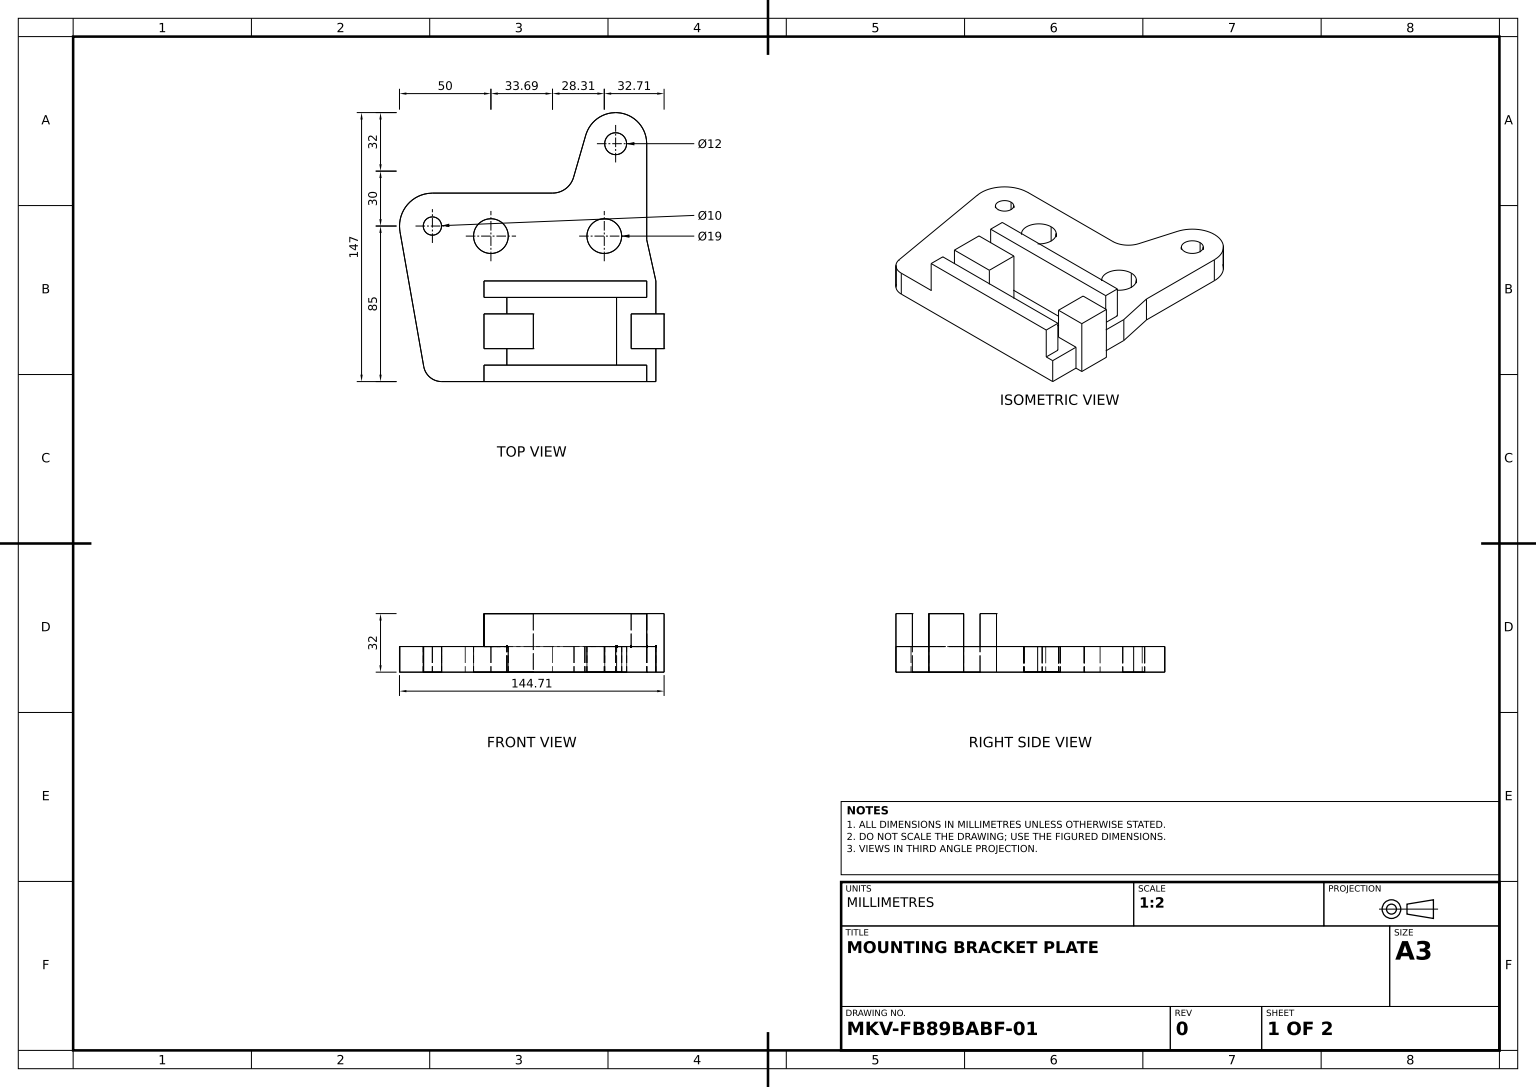
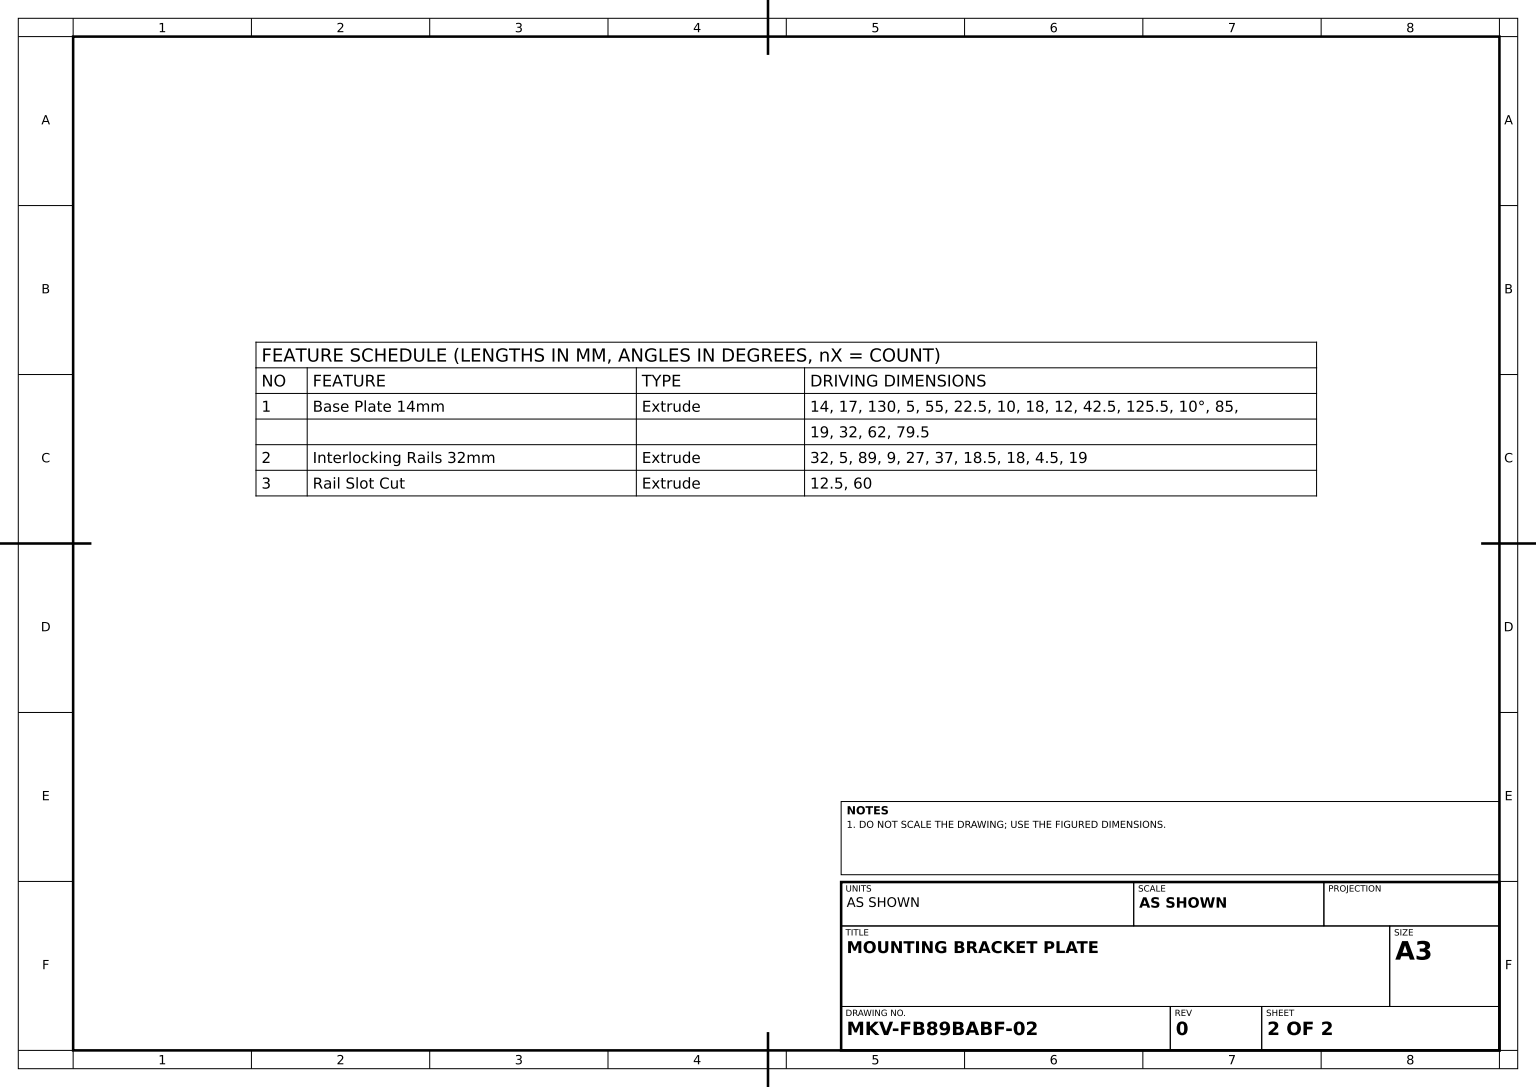
ISO-10303-21;
HEADER;
FILE_DESCRIPTION((''),'2;1');
FILE_NAME('','',(''),(''),'','','');
FILE_SCHEMA(('AUTOMOTIVE_DESIGN'));
ENDSEC;
DATA;
#1=APPLICATION_CONTEXT('');
#2=PRODUCT_CONTEXT('',#1,'mechanical');
#3=PRODUCT('','','',(#2));
#4=PRODUCT_DEFINITION_FORMATION('','',#3);
#5=PRODUCT_DEFINITION_CONTEXT('',#1,'design');
#6=PRODUCT_DEFINITION('','',#4,#5);
#7=PRODUCT_DEFINITION_SHAPE('','',#6);
#8=(LENGTH_UNIT()NAMED_UNIT(*)SI_UNIT(.MILLI.,.METRE.));
#9=(NAMED_UNIT(*)PLANE_ANGLE_UNIT()SI_UNIT($,.RADIAN.));
#10=(NAMED_UNIT(*)SI_UNIT($,.STERADIAN.)SOLID_ANGLE_UNIT());
#11=UNCERTAINTY_MEASURE_WITH_UNIT(LENGTH_MEASURE(1.E-05),#8,'distance_accuracy_value','');
#12=(GEOMETRIC_REPRESENTATION_CONTEXT(3)GLOBAL_UNCERTAINTY_ASSIGNED_CONTEXT((#11))GLOBAL_UNIT_ASSIGNED_CONTEXT((#8,#9,#10))REPRESENTATION_CONTEXT('',''));
#13=CARTESIAN_POINT('',(-67.,32.,-37.));
#14=VERTEX_POINT('',#13);
#15=CARTESIAN_POINT('',(-67.,0.,-37.));
#16=VERTEX_POINT('',#15);
#17=DIRECTION('',(0.,-1.,0.));
#18=VECTOR('',#17,1000.);
#19=LINE('',#13,#18);
#20=EDGE_CURVE('',#14,#16,#19,.T.);
#21=ORIENTED_EDGE('',*,*,#20,.T.);
#22=CARTESIAN_POINT('',(-81.5,0.,-37.));
#23=VERTEX_POINT('',#22);
#24=DIRECTION('',(-1.,0.,0.));
#25=VECTOR('',#24,1000.);
#26=LINE('',#15,#25);
#27=EDGE_CURVE('',#16,#23,#26,.T.);
#28=ORIENTED_EDGE('',*,*,#27,.T.);
#29=CARTESIAN_POINT('',(-81.5,14.,-37.));
#30=VERTEX_POINT('',#29);
#31=CARTESIAN_POINT('',(-81.5,-0.001,-37.));
#32=DIRECTION('',(0.,1.,0.));
#33=VECTOR('',#32,1000.);
#34=LINE('',#31,#33);
#35=EDGE_CURVE('',#23,#30,#34,.T.);
#36=ORIENTED_EDGE('',*,*,#35,.T.);
#37=CARTESIAN_POINT('',(-94.,14.,-37.));
#38=VERTEX_POINT('',#37);
#39=CARTESIAN_POINT('',(-22.,14.,-37.));
#40=DIRECTION('',(1.,0.,0.));
#41=VECTOR('',#40,1000.);
#42=LINE('',#39,#41);
#43=EDGE_CURVE('',#38,#30,#42,.T.);
#44=ORIENTED_EDGE('',*,*,#43,.F.);
#45=CARTESIAN_POINT('',(-94.,32.,-37.));
#46=VERTEX_POINT('',#45);
#47=LINE('',#45,#18);
#48=EDGE_CURVE('',#46,#38,#47,.T.);
#49=ORIENTED_EDGE('',*,*,#48,.F.);
#50=LINE('',#45,#25);
#51=EDGE_CURVE('',#14,#46,#50,.T.);
#52=ORIENTED_EDGE('',*,*,#51,.F.);
#53=EDGE_LOOP('',(#21,#28,#36,#44,#49,#52));
#54=FACE_OUTER_BOUND('',#53,.T.);
#55=DIRECTION('',(0.,0.,1.));
#56=AXIS2_PLACEMENT_3D('',#45,#55,#40);
#57=PLANE('',#56);
#58=ADVANCED_FACE('',(#54),#57,.F.);
#59=CARTESIAN_POINT('',(-22.,14.,-124.));
#60=VERTEX_POINT('',#59);
#61=CARTESIAN_POINT('',(-22.,14.,-136.));
#62=VERTEX_POINT('',#61);
#63=CARTESIAN_POINT('',(-22.,14.,-130.));
#64=AXIS2_PLACEMENT_3D('',#63,#32,#55);
#65=CIRCLE('',#64,6.);
#66=EDGE_CURVE('',#60,#62,#65,.T.);
#67=ORIENTED_EDGE('',*,*,#66,.T.);
#68=CARTESIAN_POINT('',(-22.,0.,-136.));
#69=VERTEX_POINT('',#68);
#70=LINE('',#61,#18);
#71=EDGE_CURVE('',#62,#69,#70,.T.);
#72=ORIENTED_EDGE('',*,*,#71,.T.);
#73=CARTESIAN_POINT('',(-22.,0.,-124.));
#74=VERTEX_POINT('',#73);
#75=CARTESIAN_POINT('',(-22.,0.,-130.));
#76=AXIS2_PLACEMENT_3D('',#75,#32,#55);
#77=CIRCLE('',#76,6.);
#78=EDGE_CURVE('',#74,#69,#77,.T.);
#79=ORIENTED_EDGE('',*,*,#78,.F.);
#80=LINE('',#59,#18);
#81=EDGE_CURVE('',#60,#74,#80,.T.);
#82=ORIENTED_EDGE('',*,*,#81,.F.);
#83=EDGE_LOOP('',(#67,#72,#79,#82));
#84=FACE_OUTER_BOUND('',#83,.T.);
#85=DIRECTION('',(0.,0.,-1.));
#86=AXIS2_PLACEMENT_3D('',#63,#17,#85);
#87=CYLINDRICAL_SURFACE('',#86,6.);
#88=ADVANCED_FACE('',(#84),#87,.F.);
#89=ORIENTED_EDGE('',*,*,#20,.F.);
#90=CARTESIAN_POINT('',(-67.,32.,-18.));
#91=VERTEX_POINT('',#90);
#92=VECTOR('',#85,1000.);
#93=LINE('',#90,#92);
#94=EDGE_CURVE('',#91,#14,#93,.T.);
#95=ORIENTED_EDGE('',*,*,#94,.F.);
#96=CARTESIAN_POINT('',(-67.,0.,-18.));
#97=VERTEX_POINT('',#96);
#98=LINE('',#90,#18);
#99=EDGE_CURVE('',#91,#97,#98,.T.);
#100=ORIENTED_EDGE('',*,*,#99,.T.);
#101=LINE('',#15,#92);
#102=EDGE_CURVE('',#97,#16,#101,.T.);
#103=ORIENTED_EDGE('',*,*,#102,.T.);
#104=EDGE_LOOP('',(#89,#95,#100,#103));
#105=FACE_OUTER_BOUND('',#104,.T.);
#106=AXIS2_PLACEMENT_3D('',#90,#24,#55);
#107=PLANE('',#106);
#108=ADVANCED_FACE('',(#105),#107,.F.);
#109=CARTESIAN_POINT('',(0.,14.,-18.));
#110=VERTEX_POINT('',#109);
#111=CARTESIAN_POINT('',(0.,0.,-18.));
#112=VERTEX_POINT('',#111);
#113=LINE('',#109,#18);
#114=EDGE_CURVE('',#110,#112,#113,.T.);
#115=ORIENTED_EDGE('',*,*,#114,.F.);
#116=CARTESIAN_POINT('',(0.,14.,0.));
#117=VERTEX_POINT('',#116);
#118=LINE('',#116,#92);
#119=EDGE_CURVE('',#117,#110,#118,.T.);
#120=ORIENTED_EDGE('',*,*,#119,.F.);
#121=CARTESIAN_POINT('',(0.,0.,0.));
#122=VERTEX_POINT('',#121);
#123=LINE('',#116,#18);
#124=EDGE_CURVE('',#117,#122,#123,.T.);
#125=ORIENTED_EDGE('',*,*,#124,.T.);
#126=LINE('',#121,#92);
#127=EDGE_CURVE('',#122,#112,#126,.T.);
#128=ORIENTED_EDGE('',*,*,#127,.T.);
#129=EDGE_LOOP('',(#115,#120,#125,#128));
#130=FACE_OUTER_BOUND('',#129,.T.);
#131=AXIS2_PLACEMENT_3D('',#116,#24,#55);
#132=PLANE('',#131);
#133=ADVANCED_FACE('',(#130),#132,.F.);
#134=CARTESIAN_POINT('',(-13.5,32.,-18.));
#135=VERTEX_POINT('',#134);
#136=CARTESIAN_POINT('',(4.5,32.,-18.));
#137=VERTEX_POINT('',#136);
#138=LINE('',#134,#41);
#139=EDGE_CURVE('',#135,#137,#138,.T.);
#140=ORIENTED_EDGE('',*,*,#139,.T.);
#141=CARTESIAN_POINT('',(4.5,32.,-37.));
#142=VERTEX_POINT('',#141);
#143=LINE('',#141,#92);
#144=EDGE_CURVE('',#137,#142,#143,.T.);
#145=ORIENTED_EDGE('',*,*,#144,.T.);
#146=CARTESIAN_POINT('',(-13.5,32.,-37.));
#147=VERTEX_POINT('',#146);
#148=LINE('',#146,#25);
#149=EDGE_CURVE('',#142,#147,#148,.T.);
#150=ORIENTED_EDGE('',*,*,#149,.T.);
#151=VECTOR('',#55,1000.);
#152=LINE('',#146,#151);
#153=EDGE_CURVE('',#147,#135,#152,.T.);
#154=ORIENTED_EDGE('',*,*,#153,.T.);
#155=EDGE_LOOP('',(#140,#145,#150,#154));
#156=FACE_OUTER_BOUND('',#155,.T.);
#157=CARTESIAN_POINT('',(0.,32.,0.));
#158=AXIS2_PLACEMENT_3D('',#157,#32,#55);
#159=PLANE('',#158);
#160=ADVANCED_FACE('',(#156),#159,.T.);
#161=ORIENTED_EDGE('',*,*,#48,.T.);
#162=CARTESIAN_POINT('',(-94.,14.,-18.));
#163=VERTEX_POINT('',#162);
#164=CARTESIAN_POINT('',(-94.,14.,-130.));
#165=LINE('',#164,#92);
#166=EDGE_CURVE('',#163,#38,#165,.T.);
#167=ORIENTED_EDGE('',*,*,#166,.F.);
#168=CARTESIAN_POINT('',(-94.,32.,-18.));
#169=VERTEX_POINT('',#168);
#170=LINE('',#168,#18);
#171=EDGE_CURVE('',#169,#163,#170,.T.);
#172=ORIENTED_EDGE('',*,*,#171,.F.);
#173=LINE('',#168,#151);
#174=EDGE_CURVE('',#46,#169,#173,.T.);
#175=ORIENTED_EDGE('',*,*,#174,.F.);
#176=EDGE_LOOP('',(#161,#167,#172,#175));
#177=FACE_OUTER_BOUND('',#176,.T.);
#178=AXIS2_PLACEMENT_3D('',#168,#40,#85);
#179=PLANE('',#178);
#180=ADVANCED_FACE('',(#177),#179,.F.);
#181=CARTESIAN_POINT('',(-44.994619,14.,-111.667904));
#182=VERTEX_POINT('',#181);
#183=CARTESIAN_POINT('',(-44.994619,0.,-111.667904));
#184=VERTEX_POINT('',#183);
#185=LINE('',#181,#18);
#186=EDGE_CURVE('',#182,#184,#185,.T.);
#187=ORIENTED_EDGE('',*,*,#186,.T.);
#188=CARTESIAN_POINT('',(-56.522721,0.,-103.));
#189=VERTEX_POINT('',#188);
#190=CARTESIAN_POINT('',(-56.522721,0.,-115.));
#191=AXIS2_PLACEMENT_3D('',#190,#17,#55);
#192=CIRCLE('',#191,12.);
#193=EDGE_CURVE('',#184,#189,#192,.T.);
#194=ORIENTED_EDGE('',*,*,#193,.T.);
#195=CARTESIAN_POINT('',(-56.522721,14.,-103.));
#196=VERTEX_POINT('',#195);
#197=LINE('',#195,#18);
#198=EDGE_CURVE('',#196,#189,#197,.T.);
#199=ORIENTED_EDGE('',*,*,#198,.F.);
#200=CARTESIAN_POINT('',(-56.522721,14.,-115.));
#201=AXIS2_PLACEMENT_3D('',#200,#17,#55);
#202=CIRCLE('',#201,12.);
#203=EDGE_CURVE('',#182,#196,#202,.T.);
#204=ORIENTED_EDGE('',*,*,#203,.F.);
#205=EDGE_LOOP('',(#187,#194,#199,#204));
#206=FACE_OUTER_BOUND('',#205,.T.);
#207=AXIS2_PLACEMENT_3D('',#200,#17,#85);
#208=CYLINDRICAL_SURFACE('',#207,12.);
#209=ADVANCED_FACE('',(#206),#208,.F.);
#210=CARTESIAN_POINT('',(-5.,32.,-55.));
#211=VERTEX_POINT('',#210);
#212=CARTESIAN_POINT('',(-5.,14.,-55.));
#213=VERTEX_POINT('',#212);
#214=LINE('',#210,#18);
#215=EDGE_CURVE('',#211,#213,#214,.T.);
#216=ORIENTED_EDGE('',*,*,#215,.F.);
#217=CARTESIAN_POINT('',(-5.,32.,-46.));
#218=VERTEX_POINT('',#217);
#219=LINE('',#217,#92);
#220=EDGE_CURVE('',#218,#211,#219,.T.);
#221=ORIENTED_EDGE('',*,*,#220,.F.);
#222=CARTESIAN_POINT('',(-5.,14.,-46.));
#223=VERTEX_POINT('',#222);
#224=LINE('',#217,#18);
#225=EDGE_CURVE('',#218,#223,#224,.T.);
#226=ORIENTED_EDGE('',*,*,#225,.T.);
#227=CARTESIAN_POINT('',(-5.,14.,-130.));
#228=LINE('',#227,#151);
#229=EDGE_CURVE('',#213,#223,#228,.T.);
#230=ORIENTED_EDGE('',*,*,#229,.F.);
#231=EDGE_LOOP('',(#216,#221,#226,#230));
#232=FACE_OUTER_BOUND('',#231,.T.);
#233=AXIS2_PLACEMENT_3D('',#217,#24,#55);
#234=PLANE('',#233);
#235=ADVANCED_FACE('',(#232),#234,.F.);
#236=CARTESIAN_POINT('',(-21.5,14.,-46.));
#237=VERTEX_POINT('',#236);
#238=CARTESIAN_POINT('',(-22.,14.,-46.));
#239=LINE('',#238,#25);
#240=EDGE_CURVE('',#223,#237,#239,.T.);
#241=ORIENTED_EDGE('',*,*,#240,.F.);
#242=ORIENTED_EDGE('',*,*,#225,.F.);
#243=CARTESIAN_POINT('',(-94.,32.,-46.));
#244=VERTEX_POINT('',#243);
#245=LINE('',#243,#41);
#246=EDGE_CURVE('',#244,#218,#245,.T.);
#247=ORIENTED_EDGE('',*,*,#246,.F.);
#248=CARTESIAN_POINT('',(-94.,14.,-46.));
#249=VERTEX_POINT('',#248);
#250=LINE('',#243,#18);
#251=EDGE_CURVE('',#244,#249,#250,.T.);
#252=ORIENTED_EDGE('',*,*,#251,.T.);
#253=CARTESIAN_POINT('',(-81.5,14.,-46.));
#254=VERTEX_POINT('',#253);
#255=EDGE_CURVE('',#254,#249,#239,.T.);
#256=ORIENTED_EDGE('',*,*,#255,.F.);
#257=CARTESIAN_POINT('',(-81.5,0.,-46.));
#258=VERTEX_POINT('',#257);
#259=CARTESIAN_POINT('',(-81.5,-0.001,-46.));
#260=LINE('',#259,#33);
#261=EDGE_CURVE('',#258,#254,#260,.T.);
#262=ORIENTED_EDGE('',*,*,#261,.F.);
#263=CARTESIAN_POINT('',(-21.5,0.,-46.));
#264=VERTEX_POINT('',#263);
#265=LINE('',#257,#41);
#266=EDGE_CURVE('',#258,#264,#265,.T.);
#267=ORIENTED_EDGE('',*,*,#266,.T.);
#268=CARTESIAN_POINT('',(-21.5,-0.001,-46.));
#269=LINE('',#268,#33);
#270=EDGE_CURVE('',#264,#237,#269,.T.);
#271=ORIENTED_EDGE('',*,*,#270,.T.);
#272=EDGE_LOOP('',(#241,#242,#247,#252,#256,#262,#267,#271));
#273=FACE_OUTER_BOUND('',#272,.T.);
#274=AXIS2_PLACEMENT_3D('',#243,#85,#24);
#275=PLANE('',#274);
#276=ADVANCED_FACE('',(#273),#275,.F.);
#277=CARTESIAN_POINT('',(-90.210114,0.,-70.));
#278=VERTEX_POINT('',#277);
#279=CARTESIAN_POINT('',(-90.210114,0.,-89.));
#280=VERTEX_POINT('',#279);
#281=CARTESIAN_POINT('',(-90.210114,0.,-79.5));
#282=AXIS2_PLACEMENT_3D('',#281,#32,#55);
#283=CIRCLE('',#282,9.5);
#284=EDGE_CURVE('',#278,#280,#283,.T.);
#285=ORIENTED_EDGE('',*,*,#284,.F.);
#286=CARTESIAN_POINT('',(-90.210114,14.,-70.));
#287=VERTEX_POINT('',#286);
#288=LINE('',#286,#18);
#289=EDGE_CURVE('',#287,#278,#288,.T.);
#290=ORIENTED_EDGE('',*,*,#289,.F.);
#291=CARTESIAN_POINT('',(-90.210114,14.,-89.));
#292=VERTEX_POINT('',#291);
#293=CARTESIAN_POINT('',(-90.210114,14.,-79.5));
#294=AXIS2_PLACEMENT_3D('',#293,#32,#55);
#295=CIRCLE('',#294,9.5);
#296=EDGE_CURVE('',#287,#292,#295,.T.);
#297=ORIENTED_EDGE('',*,*,#296,.T.);
#298=LINE('',#291,#18);
#299=EDGE_CURVE('',#292,#280,#298,.T.);
#300=ORIENTED_EDGE('',*,*,#299,.T.);
#301=EDGE_LOOP('',(#285,#290,#297,#300));
#302=FACE_OUTER_BOUND('',#301,.T.);
#303=AXIS2_PLACEMENT_3D('',#293,#17,#85);
#304=CYLINDRICAL_SURFACE('',#303,9.5);
#305=ADVANCED_FACE('',(#302),#304,.F.);
#306=CARTESIAN_POINT('',(-5.,14.,-77.5));
#307=VERTEX_POINT('',#306);
#308=VERTEX_POINT('',#227);
#309=LINE('',#306,#92);
#310=EDGE_CURVE('',#307,#308,#309,.T.);
#311=ORIENTED_EDGE('',*,*,#310,.F.);
#312=CARTESIAN_POINT('',(-5.,0.,-77.5));
#313=VERTEX_POINT('',#312);
#314=LINE('',#306,#18);
#315=EDGE_CURVE('',#307,#313,#314,.T.);
#316=ORIENTED_EDGE('',*,*,#315,.T.);
#317=CARTESIAN_POINT('',(-5.,0.,-130.));
#318=VERTEX_POINT('',#317);
#319=LINE('',#312,#92);
#320=EDGE_CURVE('',#313,#318,#319,.T.);
#321=ORIENTED_EDGE('',*,*,#320,.T.);
#322=LINE('',#227,#18);
#323=EDGE_CURVE('',#308,#318,#322,.T.);
#324=ORIENTED_EDGE('',*,*,#323,.F.);
#325=EDGE_LOOP('',(#311,#316,#321,#324));
#326=FACE_OUTER_BOUND('',#325,.T.);
#327=AXIS2_PLACEMENT_3D('',#306,#24,#55);
#328=PLANE('',#327);
#329=ADVANCED_FACE('',(#326),#328,.F.);
#330=CARTESIAN_POINT('',(-21.5,0.,-9.));
#331=VERTEX_POINT('',#330);
#332=CARTESIAN_POINT('',(-21.5,14.,-9.));
#333=VERTEX_POINT('',#332);
#334=CARTESIAN_POINT('',(-21.5,-0.001,-9.));
#335=LINE('',#334,#33);
#336=EDGE_CURVE('',#331,#333,#335,.T.);
#337=ORIENTED_EDGE('',*,*,#336,.T.);
#338=LINE('',#236,#92);
#339=EDGE_CURVE('',#333,#237,#338,.T.);
#340=ORIENTED_EDGE('',*,*,#339,.T.);
#341=ORIENTED_EDGE('',*,*,#270,.F.);
#342=LINE('',#263,#151);
#343=EDGE_CURVE('',#264,#331,#342,.T.);
#344=ORIENTED_EDGE('',*,*,#343,.T.);
#345=EDGE_LOOP('',(#337,#340,#341,#344));
#346=FACE_OUTER_BOUND('',#345,.T.);
#347=AXIS2_PLACEMENT_3D('',#268,#40,#85);
#348=PLANE('',#347);
#349=ADVANCED_FACE('',(#346),#348,.F.);
#350=CARTESIAN_POINT('',(-122.210114,14.,-90.));
#351=VERTEX_POINT('',#350);
#352=CARTESIAN_POINT('',(-122.210114,0.,-90.));
#353=VERTEX_POINT('',#352);
#354=LINE('',#350,#18);
#355=EDGE_CURVE('',#351,#353,#354,.T.);
#356=ORIENTED_EDGE('',*,*,#355,.T.);
#357=CARTESIAN_POINT('',(-122.210114,0.,-80.));
#358=VERTEX_POINT('',#357);
#359=CARTESIAN_POINT('',(-122.210114,0.,-85.));
#360=AXIS2_PLACEMENT_3D('',#359,#32,#55);
#361=CIRCLE('',#360,5.);
#362=EDGE_CURVE('',#358,#353,#361,.T.);
#363=ORIENTED_EDGE('',*,*,#362,.F.);
#364=CARTESIAN_POINT('',(-122.210114,14.,-80.));
#365=VERTEX_POINT('',#364);
#366=LINE('',#364,#18);
#367=EDGE_CURVE('',#365,#358,#366,.T.);
#368=ORIENTED_EDGE('',*,*,#367,.F.);
#369=CARTESIAN_POINT('',(-122.210114,14.,-85.));
#370=AXIS2_PLACEMENT_3D('',#369,#32,#55);
#371=CIRCLE('',#370,5.);
#372=EDGE_CURVE('',#365,#351,#371,.T.);
#373=ORIENTED_EDGE('',*,*,#372,.T.);
#374=EDGE_LOOP('',(#356,#363,#368,#373));
#375=FACE_OUTER_BOUND('',#374,.T.);
#376=AXIS2_PLACEMENT_3D('',#369,#17,#85);
#377=CYLINDRICAL_SURFACE('',#376,5.);
#378=ADVANCED_FACE('',(#375),#377,.F.);
#379=CARTESIAN_POINT('',(-13.5,14.,-18.));
#380=VERTEX_POINT('',#379);
#381=LINE('',#134,#18);
#382=EDGE_CURVE('',#135,#380,#381,.T.);
#383=ORIENTED_EDGE('',*,*,#382,.T.);
#384=CARTESIAN_POINT('',(-22.,14.,-18.));
#385=LINE('',#384,#25);
#386=EDGE_CURVE('',#110,#380,#385,.T.);
#387=ORIENTED_EDGE('',*,*,#386,.F.);
#388=ORIENTED_EDGE('',*,*,#114,.T.);
#389=CARTESIAN_POINT('',(4.5,0.,-18.));
#390=VERTEX_POINT('',#389);
#391=CARTESIAN_POINT('',(-13.5,0.,-18.));
#392=LINE('',#391,#41);
#393=EDGE_CURVE('',#112,#390,#392,.T.);
#394=ORIENTED_EDGE('',*,*,#393,.T.);
#395=LINE('',#136,#18);
#396=EDGE_CURVE('',#137,#390,#395,.T.);
#397=ORIENTED_EDGE('',*,*,#396,.F.);
#398=ORIENTED_EDGE('',*,*,#139,.F.);
#399=EDGE_LOOP('',(#383,#387,#388,#394,#397,#398));
#400=FACE_OUTER_BOUND('',#399,.T.);
#401=AXIS2_PLACEMENT_3D('',#134,#85,#24);
#402=PLANE('',#401);
#403=ADVANCED_FACE('',(#400),#402,.F.);
#404=ORIENTED_EDGE('',*,*,#171,.T.);
#405=CARTESIAN_POINT('',(-81.5,14.,-18.));
#406=VERTEX_POINT('',#405);
#407=EDGE_CURVE('',#406,#163,#385,.T.);
#408=ORIENTED_EDGE('',*,*,#407,.F.);
#409=CARTESIAN_POINT('',(-81.5,0.,-18.));
#410=VERTEX_POINT('',#409);
#411=CARTESIAN_POINT('',(-81.5,-0.001,-18.));
#412=LINE('',#411,#33);
#413=EDGE_CURVE('',#410,#406,#412,.T.);
#414=ORIENTED_EDGE('',*,*,#413,.F.);
#415=LINE('',#96,#41);
#416=EDGE_CURVE('',#410,#97,#415,.T.);
#417=ORIENTED_EDGE('',*,*,#416,.T.);
#418=ORIENTED_EDGE('',*,*,#99,.F.);
#419=LINE('',#168,#41);
#420=EDGE_CURVE('',#169,#91,#419,.T.);
#421=ORIENTED_EDGE('',*,*,#420,.F.);
#422=EDGE_LOOP('',(#404,#408,#414,#417,#418,#421));
#423=FACE_OUTER_BOUND('',#422,.T.);
#424=AXIS2_PLACEMENT_3D('',#168,#85,#24);
#425=PLANE('',#424);
#426=ADVANCED_FACE('',(#423),#425,.F.);
#427=CARTESIAN_POINT('',(-5.,32.,0.));
#428=VERTEX_POINT('',#427);
#429=CARTESIAN_POINT('',(-5.,32.,-9.));
#430=VERTEX_POINT('',#429);
#431=LINE('',#427,#92);
#432=EDGE_CURVE('',#428,#430,#431,.T.);
#433=ORIENTED_EDGE('',*,*,#432,.T.);
#434=CARTESIAN_POINT('',(-94.,32.,-9.));
#435=VERTEX_POINT('',#434);
#436=LINE('',#434,#25);
#437=EDGE_CURVE('',#430,#435,#436,.T.);
#438=ORIENTED_EDGE('',*,*,#437,.T.);
#439=CARTESIAN_POINT('',(-94.,32.,0.));
#440=VERTEX_POINT('',#439);
#441=LINE('',#439,#151);
#442=EDGE_CURVE('',#435,#440,#441,.T.);
#443=ORIENTED_EDGE('',*,*,#442,.T.);
#444=LINE('',#439,#41);
#445=EDGE_CURVE('',#440,#428,#444,.T.);
#446=ORIENTED_EDGE('',*,*,#445,.T.);
#447=EDGE_LOOP('',(#433,#438,#443,#446));
#448=FACE_OUTER_BOUND('',#447,.T.);
#449=AXIS2_PLACEMENT_3D('',#157,#17,#85);
#450=PLANE('',#449);
#451=ADVANCED_FACE('',(#448),#450,.F.);
#452=CARTESIAN_POINT('',(-13.5,14.,-37.));
#453=VERTEX_POINT('',#452);
#454=LINE('',#146,#18);
#455=EDGE_CURVE('',#147,#453,#454,.T.);
#456=ORIENTED_EDGE('',*,*,#455,.T.);
#457=CARTESIAN_POINT('',(-13.5,14.,-130.));
#458=LINE('',#457,#92);
#459=EDGE_CURVE('',#380,#453,#458,.T.);
#460=ORIENTED_EDGE('',*,*,#459,.F.);
#461=ORIENTED_EDGE('',*,*,#382,.F.);
#462=ORIENTED_EDGE('',*,*,#153,.F.);
#463=EDGE_LOOP('',(#456,#460,#461,#462));
#464=FACE_OUTER_BOUND('',#463,.T.);
#465=AXIS2_PLACEMENT_3D('',#146,#40,#85);
#466=PLANE('',#465);
#467=ADVANCED_FACE('',(#464),#466,.F.);
#468=CARTESIAN_POINT('',(-126.957081,14.,-8.263518));
#469=VERTEX_POINT('',#468);
#470=CARTESIAN_POINT('',(-117.109004,14.,0.));
#471=VERTEX_POINT('',#470);
#472=CARTESIAN_POINT('',(-117.109004,14.,-10.));
#473=AXIS2_PLACEMENT_3D('',#472,#32,#85);
#474=CIRCLE('',#473,10.);
#475=EDGE_CURVE('',#469,#471,#474,.T.);
#476=ORIENTED_EDGE('',*,*,#475,.F.);
#477=CARTESIAN_POINT('',(-126.957081,0.,-8.263518));
#478=VERTEX_POINT('',#477);
#479=LINE('',#468,#18);
#480=EDGE_CURVE('',#469,#478,#479,.T.);
#481=ORIENTED_EDGE('',*,*,#480,.T.);
#482=CARTESIAN_POINT('',(-117.109004,0.,0.));
#483=VERTEX_POINT('',#482);
#484=CARTESIAN_POINT('',(-117.109004,0.,-10.));
#485=AXIS2_PLACEMENT_3D('',#484,#32,#85);
#486=CIRCLE('',#485,10.);
#487=EDGE_CURVE('',#478,#483,#486,.T.);
#488=ORIENTED_EDGE('',*,*,#487,.T.);
#489=LINE('',#470,#18);
#490=EDGE_CURVE('',#471,#483,#489,.T.);
#491=ORIENTED_EDGE('',*,*,#490,.F.);
#492=EDGE_LOOP('',(#476,#481,#488,#491));
#493=FACE_OUTER_BOUND('',#492,.T.);
#494=AXIS2_PLACEMENT_3D('',#472,#17,#85);
#495=CYLINDRICAL_SURFACE('',#494,10.);
#496=ADVANCED_FACE('',(#493),#495,.T.);
#497=CARTESIAN_POINT('',(-94.,14.,-9.));
#498=VERTEX_POINT('',#497);
#499=LINE('',#434,#18);
#500=EDGE_CURVE('',#435,#498,#499,.T.);
#501=ORIENTED_EDGE('',*,*,#500,.F.);
#502=ORIENTED_EDGE('',*,*,#437,.F.);
#503=CARTESIAN_POINT('',(-5.,14.,-9.));
#504=VERTEX_POINT('',#503);
#505=LINE('',#429,#18);
#506=EDGE_CURVE('',#430,#504,#505,.T.);
#507=ORIENTED_EDGE('',*,*,#506,.T.);
#508=CARTESIAN_POINT('',(-22.,14.,-9.));
#509=LINE('',#508,#41);
#510=EDGE_CURVE('',#333,#504,#509,.T.);
#511=ORIENTED_EDGE('',*,*,#510,.F.);
#512=ORIENTED_EDGE('',*,*,#336,.F.);
#513=CARTESIAN_POINT('',(-81.5,0.,-9.));
#514=VERTEX_POINT('',#513);
#515=LINE('',#513,#25);
#516=EDGE_CURVE('',#331,#514,#515,.T.);
#517=ORIENTED_EDGE('',*,*,#516,.T.);
#518=CARTESIAN_POINT('',(-81.5,14.,-9.));
#519=VERTEX_POINT('',#518);
#520=CARTESIAN_POINT('',(-81.5,-0.001,-9.));
#521=LINE('',#520,#33);
#522=EDGE_CURVE('',#514,#519,#521,.T.);
#523=ORIENTED_EDGE('',*,*,#522,.T.);
#524=EDGE_CURVE('',#498,#519,#509,.T.);
#525=ORIENTED_EDGE('',*,*,#524,.F.);
#526=EDGE_LOOP('',(#501,#502,#507,#511,#512,#517,#523,#525));
#527=FACE_OUTER_BOUND('',#526,.T.);
#528=AXIS2_PLACEMENT_3D('',#434,#55,#40);
#529=PLANE('',#528);
#530=ADVANCED_FACE('',(#527),#529,.F.);
#531=ORIENTED_EDGE('',*,*,#94,.T.);
#532=ORIENTED_EDGE('',*,*,#51,.T.);
#533=ORIENTED_EDGE('',*,*,#174,.T.);
#534=ORIENTED_EDGE('',*,*,#420,.T.);
#535=EDGE_LOOP('',(#531,#532,#533,#534));
#536=FACE_OUTER_BOUND('',#535,.T.);
#537=ADVANCED_FACE('',(#536),#450,.F.);
#538=ORIENTED_EDGE('',*,*,#455,.F.);
#539=ORIENTED_EDGE('',*,*,#149,.F.);
#540=CARTESIAN_POINT('',(4.5,0.,-37.));
#541=VERTEX_POINT('',#540);
#542=LINE('',#141,#18);
#543=EDGE_CURVE('',#142,#541,#542,.T.);
#544=ORIENTED_EDGE('',*,*,#543,.T.);
#545=CARTESIAN_POINT('',(0.,0.,-37.));
#546=VERTEX_POINT('',#545);
#547=CARTESIAN_POINT('',(-13.5,0.,-37.));
#548=LINE('',#547,#25);
#549=EDGE_CURVE('',#541,#546,#548,.T.);
#550=ORIENTED_EDGE('',*,*,#549,.T.);
#551=CARTESIAN_POINT('',(0.,14.,-37.));
#552=VERTEX_POINT('',#551);
#553=LINE('',#551,#33);
#554=EDGE_CURVE('',#546,#552,#553,.T.);
#555=ORIENTED_EDGE('',*,*,#554,.T.);
#556=EDGE_CURVE('',#453,#552,#42,.T.);
#557=ORIENTED_EDGE('',*,*,#556,.F.);
#558=EDGE_LOOP('',(#538,#539,#544,#550,#555,#557));
#559=FACE_OUTER_BOUND('',#558,.T.);
#560=AXIS2_PLACEMENT_3D('',#146,#55,#40);
#561=PLANE('',#560);
#562=ADVANCED_FACE('',(#559),#561,.F.);
#563=CARTESIAN_POINT('',(-28.210114,0.,-89.));
#564=VERTEX_POINT('',#563);
#565=CARTESIAN_POINT('',(-28.210114,0.,-70.));
#566=VERTEX_POINT('',#565);
#567=CARTESIAN_POINT('',(-28.210114,0.,-79.5));
#568=AXIS2_PLACEMENT_3D('',#567,#32,#55);
#569=CIRCLE('',#568,9.5);
#570=EDGE_CURVE('',#564,#566,#569,.T.);
#571=ORIENTED_EDGE('',*,*,#570,.F.);
#572=CARTESIAN_POINT('',(-28.210114,14.,-89.));
#573=VERTEX_POINT('',#572);
#574=LINE('',#572,#18);
#575=EDGE_CURVE('',#573,#564,#574,.T.);
#576=ORIENTED_EDGE('',*,*,#575,.F.);
#577=CARTESIAN_POINT('',(-28.210114,14.,-70.));
#578=VERTEX_POINT('',#577);
#579=CARTESIAN_POINT('',(-28.210114,14.,-79.5));
#580=AXIS2_PLACEMENT_3D('',#579,#32,#55);
#581=CIRCLE('',#580,9.5);
#582=EDGE_CURVE('',#573,#578,#581,.T.);
#583=ORIENTED_EDGE('',*,*,#582,.T.);
#584=LINE('',#577,#18);
#585=EDGE_CURVE('',#578,#566,#584,.T.);
#586=ORIENTED_EDGE('',*,*,#585,.T.);
#587=EDGE_LOOP('',(#571,#576,#583,#586));
#588=FACE_OUTER_BOUND('',#587,.T.);
#589=AXIS2_PLACEMENT_3D('',#579,#17,#85);
#590=CYLINDRICAL_SURFACE('',#589,9.5);
#591=ADVANCED_FACE('',(#588),#590,.F.);
#592=CARTESIAN_POINT('',(-139.936654,14.,-81.874333));
#593=VERTEX_POINT('',#592);
#594=CARTESIAN_POINT('',(-139.936654,0.,-81.874333));
#595=VERTEX_POINT('',#594);
#596=LINE('',#592,#18);
#597=EDGE_CURVE('',#593,#595,#596,.T.);
#598=ORIENTED_EDGE('',*,*,#597,.F.);
#599=CARTESIAN_POINT('',(-122.210114,14.,-103.));
#600=VERTEX_POINT('',#599);
#601=AXIS2_PLACEMENT_3D('',#369,#32,#85);
#602=CIRCLE('',#601,18.);
#603=EDGE_CURVE('',#600,#593,#602,.T.);
#604=ORIENTED_EDGE('',*,*,#603,.F.);
#605=CARTESIAN_POINT('',(-122.210114,0.,-103.));
#606=VERTEX_POINT('',#605);
#607=LINE('',#599,#18);
#608=EDGE_CURVE('',#600,#606,#607,.T.);
#609=ORIENTED_EDGE('',*,*,#608,.T.);
#610=AXIS2_PLACEMENT_3D('',#359,#32,#85);
#611=CIRCLE('',#610,18.);
#612=EDGE_CURVE('',#606,#595,#611,.T.);
#613=ORIENTED_EDGE('',*,*,#612,.T.);
#614=EDGE_LOOP('',(#598,#604,#609,#613));
#615=FACE_OUTER_BOUND('',#614,.T.);
#616=CYLINDRICAL_SURFACE('',#376,18.);
#617=ADVANCED_FACE('',(#615),#616,.T.);
#618=ORIENTED_EDGE('',*,*,#597,.T.);
#619=DIRECTION('',(0.173648178,0.,0.984807753));
#620=VECTOR('',#619,1000.);
#621=LINE('',#477,#620);
#622=EDGE_CURVE('',#595,#478,#621,.T.);
#623=ORIENTED_EDGE('',*,*,#622,.T.);
#624=ORIENTED_EDGE('',*,*,#480,.F.);
#625=LINE('',#468,#620);
#626=EDGE_CURVE('',#593,#469,#625,.T.);
#627=ORIENTED_EDGE('',*,*,#626,.F.);
#628=EDGE_LOOP('',(#618,#623,#624,#627));
#629=FACE_OUTER_BOUND('',#628,.T.);
#630=DIRECTION('',(0.984807753,0.,-0.173648178));
#631=DIRECTION('',(-0.173648178,0.,-0.984807753));
#632=AXIS2_PLACEMENT_3D('',#468,#630,#631);
#633=PLANE('',#632);
#634=ADVANCED_FACE('',(#629),#633,.F.);
#635=CARTESIAN_POINT('',(-94.,32.,-55.));
#636=VERTEX_POINT('',#635);
#637=LINE('',#635,#25);
#638=EDGE_CURVE('',#211,#636,#637,.T.);
#639=ORIENTED_EDGE('',*,*,#638,.F.);
#640=ORIENTED_EDGE('',*,*,#215,.T.);
#641=CARTESIAN_POINT('',(-94.,14.,-55.));
#642=VERTEX_POINT('',#641);
#643=CARTESIAN_POINT('',(-22.,14.,-55.));
#644=LINE('',#643,#41);
#645=EDGE_CURVE('',#642,#213,#644,.T.);
#646=ORIENTED_EDGE('',*,*,#645,.F.);
#647=LINE('',#635,#18);
#648=EDGE_CURVE('',#636,#642,#647,.T.);
#649=ORIENTED_EDGE('',*,*,#648,.F.);
#650=EDGE_LOOP('',(#639,#640,#646,#649));
#651=FACE_OUTER_BOUND('',#650,.T.);
#652=AXIS2_PLACEMENT_3D('',#635,#55,#40);
#653=PLANE('',#652);
#654=ADVANCED_FACE('',(#651),#653,.F.);
#655=EDGE_CURVE('',#280,#278,#283,.T.);
#656=ORIENTED_EDGE('',*,*,#655,.T.);
#657=ORIENTED_EDGE('',*,*,#284,.T.);
#658=EDGE_LOOP('',(#656,#657));
#659=FACE_BOUND('',#658,.T.);
#660=ORIENTED_EDGE('',*,*,#393,.F.);
#661=ORIENTED_EDGE('',*,*,#127,.F.);
#662=LINE('',#121,#41);
#663=EDGE_CURVE('',#483,#122,#662,.T.);
#664=ORIENTED_EDGE('',*,*,#663,.F.);
#665=ORIENTED_EDGE('',*,*,#487,.F.);
#666=ORIENTED_EDGE('',*,*,#622,.F.);
#667=ORIENTED_EDGE('',*,*,#612,.F.);
#668=LINE('',#605,#25);
#669=EDGE_CURVE('',#189,#606,#668,.T.);
#670=ORIENTED_EDGE('',*,*,#669,.F.);
#671=ORIENTED_EDGE('',*,*,#193,.F.);
#672=CARTESIAN_POINT('',(-38.331478,0.,-134.72047));
#673=VERTEX_POINT('',#672);
#674=DIRECTION('',(-0.27767469,0.,0.960675162));
#675=VECTOR('',#674,1000.);
#676=LINE('',#183,#675);
#677=EDGE_CURVE('',#673,#184,#676,.T.);
#678=ORIENTED_EDGE('',*,*,#677,.F.);
#679=CARTESIAN_POINT('',(-22.,0.,-147.));
#680=VERTEX_POINT('',#679);
#681=CIRCLE('',#76,17.);
#682=EDGE_CURVE('',#680,#673,#681,.T.);
#683=ORIENTED_EDGE('',*,*,#682,.F.);
#684=EDGE_CURVE('',#318,#680,#681,.T.);
#685=ORIENTED_EDGE('',*,*,#684,.F.);
#686=ORIENTED_EDGE('',*,*,#320,.F.);
#687=CARTESIAN_POINT('',(0.,0.,-55.));
#688=VERTEX_POINT('',#687);
#689=DIRECTION('',(-0.216930458,0.,-0.97618706));
#690=VECTOR('',#689,1000.);
#691=LINE('',#687,#690);
#692=EDGE_CURVE('',#688,#313,#691,.T.);
#693=ORIENTED_EDGE('',*,*,#692,.F.);
#694=EDGE_CURVE('',#546,#688,#126,.T.);
#695=ORIENTED_EDGE('',*,*,#694,.F.);
#696=ORIENTED_EDGE('',*,*,#549,.F.);
#697=LINE('',#540,#92);
#698=EDGE_CURVE('',#390,#541,#697,.T.);
#699=ORIENTED_EDGE('',*,*,#698,.F.);
#700=EDGE_LOOP('',(#660,#661,#664,#665,#666,#667,#670,#671,#678,#683,#685,#686,#693,#695,#696,#699));
#701=FACE_OUTER_BOUND('',#700,.T.);
#702=ORIENTED_EDGE('',*,*,#78,.T.);
#703=EDGE_CURVE('',#69,#74,#77,.T.);
#704=ORIENTED_EDGE('',*,*,#703,.T.);
#705=EDGE_LOOP('',(#702,#704));
#706=FACE_BOUND('',#705,.T.);
#707=ORIENTED_EDGE('',*,*,#570,.T.);
#708=EDGE_CURVE('',#566,#564,#569,.T.);
#709=ORIENTED_EDGE('',*,*,#708,.T.);
#710=EDGE_LOOP('',(#707,#709));
#711=FACE_BOUND('',#710,.T.);
#712=ORIENTED_EDGE('',*,*,#102,.F.);
#713=ORIENTED_EDGE('',*,*,#416,.F.);
#714=LINE('',#409,#92);
#715=EDGE_CURVE('',#514,#410,#714,.T.);
#716=ORIENTED_EDGE('',*,*,#715,.F.);
#717=ORIENTED_EDGE('',*,*,#516,.F.);
#718=ORIENTED_EDGE('',*,*,#343,.F.);
#719=ORIENTED_EDGE('',*,*,#266,.F.);
#720=LINE('',#257,#92);
#721=EDGE_CURVE('',#23,#258,#720,.T.);
#722=ORIENTED_EDGE('',*,*,#721,.F.);
#723=ORIENTED_EDGE('',*,*,#27,.F.);
#724=EDGE_LOOP('',(#712,#713,#716,#717,#718,#719,#722,#723));
#725=FACE_BOUND('',#724,.T.);
#726=EDGE_CURVE('',#353,#358,#361,.T.);
#727=ORIENTED_EDGE('',*,*,#726,.T.);
#728=ORIENTED_EDGE('',*,*,#362,.T.);
#729=EDGE_LOOP('',(#727,#728));
#730=FACE_BOUND('',#729,.T.);
#731=PLANE('',#76);
#732=ADVANCED_FACE('',(#659,#701,#706,#711,#725,#730),#731,.F.);
#733=ORIENTED_EDGE('',*,*,#144,.F.);
#734=ORIENTED_EDGE('',*,*,#396,.T.);
#735=ORIENTED_EDGE('',*,*,#698,.T.);
#736=ORIENTED_EDGE('',*,*,#543,.F.);
#737=EDGE_LOOP('',(#733,#734,#735,#736));
#738=FACE_OUTER_BOUND('',#737,.T.);
#739=AXIS2_PLACEMENT_3D('',#141,#24,#55);
#740=PLANE('',#739);
#741=ADVANCED_FACE('',(#738),#740,.F.);
#742=ORIENTED_EDGE('',*,*,#648,.T.);
#743=EDGE_CURVE('',#249,#642,#165,.T.);
#744=ORIENTED_EDGE('',*,*,#743,.F.);
#745=ORIENTED_EDGE('',*,*,#251,.F.);
#746=LINE('',#243,#151);
#747=EDGE_CURVE('',#636,#244,#746,.T.);
#748=ORIENTED_EDGE('',*,*,#747,.F.);
#749=EDGE_LOOP('',(#742,#744,#745,#748));
#750=FACE_OUTER_BOUND('',#749,.T.);
#751=AXIS2_PLACEMENT_3D('',#243,#40,#85);
#752=PLANE('',#751);
#753=ADVANCED_FACE('',(#750),#752,.F.);
#754=CARTESIAN_POINT('',(0.,14.,-55.));
#755=VERTEX_POINT('',#754);
#756=EDGE_CURVE('',#552,#755,#118,.T.);
#757=ORIENTED_EDGE('',*,*,#756,.F.);
#758=ORIENTED_EDGE('',*,*,#554,.F.);
#759=ORIENTED_EDGE('',*,*,#694,.T.);
#760=LINE('',#754,#18);
#761=EDGE_CURVE('',#755,#688,#760,.T.);
#762=ORIENTED_EDGE('',*,*,#761,.F.);
#763=EDGE_LOOP('',(#757,#758,#759,#762));
#764=FACE_OUTER_BOUND('',#763,.T.);
#765=ADVANCED_FACE('',(#764),#132,.F.);
#766=CARTESIAN_POINT('',(-5.,14.,0.));
#767=VERTEX_POINT('',#766);
#768=EDGE_CURVE('',#504,#767,#228,.T.);
#769=ORIENTED_EDGE('',*,*,#768,.F.);
#770=ORIENTED_EDGE('',*,*,#506,.F.);
#771=ORIENTED_EDGE('',*,*,#432,.F.);
#772=LINE('',#427,#18);
#773=EDGE_CURVE('',#428,#767,#772,.T.);
#774=ORIENTED_EDGE('',*,*,#773,.T.);
#775=EDGE_LOOP('',(#769,#770,#771,#774));
#776=FACE_OUTER_BOUND('',#775,.T.);
#777=AXIS2_PLACEMENT_3D('',#427,#24,#55);
#778=PLANE('',#777);
#779=ADVANCED_FACE('',(#776),#778,.F.);
#780=ORIENTED_EDGE('',*,*,#81,.T.);
#781=ORIENTED_EDGE('',*,*,#703,.F.);
#782=ORIENTED_EDGE('',*,*,#71,.F.);
#783=EDGE_CURVE('',#62,#60,#65,.T.);
#784=ORIENTED_EDGE('',*,*,#783,.T.);
#785=EDGE_LOOP('',(#780,#781,#782,#784));
#786=FACE_OUTER_BOUND('',#785,.T.);
#787=ADVANCED_FACE('',(#786),#87,.F.);
#788=ORIENTED_EDGE('',*,*,#522,.F.);
#789=ORIENTED_EDGE('',*,*,#715,.T.);
#790=ORIENTED_EDGE('',*,*,#413,.T.);
#791=LINE('',#405,#151);
#792=EDGE_CURVE('',#406,#519,#791,.T.);
#793=ORIENTED_EDGE('',*,*,#792,.T.);
#794=EDGE_LOOP('',(#788,#789,#790,#793));
#795=FACE_OUTER_BOUND('',#794,.T.);
#796=AXIS2_PLACEMENT_3D('',#411,#24,#55);
#797=PLANE('',#796);
#798=ADVANCED_FACE('',(#795),#797,.F.);
#799=CARTESIAN_POINT('',(-38.331478,14.,-134.72047));
#800=VERTEX_POINT('',#799);
#801=LINE('',#799,#18);
#802=EDGE_CURVE('',#800,#673,#801,.T.);
#803=ORIENTED_EDGE('',*,*,#802,.T.);
#804=ORIENTED_EDGE('',*,*,#677,.T.);
#805=ORIENTED_EDGE('',*,*,#186,.F.);
#806=LINE('',#181,#675);
#807=EDGE_CURVE('',#800,#182,#806,.T.);
#808=ORIENTED_EDGE('',*,*,#807,.F.);
#809=EDGE_LOOP('',(#803,#804,#805,#808));
#810=FACE_OUTER_BOUND('',#809,.T.);
#811=DIRECTION('',(0.960675162,0.,0.27767469));
#812=DIRECTION('',(0.27767469,0.,-0.960675162));
#813=AXIS2_PLACEMENT_3D('',#181,#811,#812);
#814=PLANE('',#813);
#815=ADVANCED_FACE('',(#810),#814,.F.);
#816=ORIENTED_EDGE('',*,*,#556,.T.);
#817=ORIENTED_EDGE('',*,*,#756,.T.);
#818=LINE('',#754,#690);
#819=EDGE_CURVE('',#755,#307,#818,.T.);
#820=ORIENTED_EDGE('',*,*,#819,.T.);
#821=ORIENTED_EDGE('',*,*,#310,.T.);
#822=CARTESIAN_POINT('',(-22.,14.,-147.));
#823=VERTEX_POINT('',#822);
#824=CIRCLE('',#64,17.);
#825=EDGE_CURVE('',#308,#823,#824,.T.);
#826=ORIENTED_EDGE('',*,*,#825,.T.);
#827=EDGE_CURVE('',#823,#800,#824,.T.);
#828=ORIENTED_EDGE('',*,*,#827,.T.);
#829=ORIENTED_EDGE('',*,*,#807,.T.);
#830=ORIENTED_EDGE('',*,*,#203,.T.);
#831=LINE('',#599,#25);
#832=EDGE_CURVE('',#196,#600,#831,.T.);
#833=ORIENTED_EDGE('',*,*,#832,.T.);
#834=ORIENTED_EDGE('',*,*,#603,.T.);
#835=ORIENTED_EDGE('',*,*,#626,.T.);
#836=ORIENTED_EDGE('',*,*,#475,.T.);
#837=CARTESIAN_POINT('',(-94.,14.,0.));
#838=VERTEX_POINT('',#837);
#839=LINE('',#116,#41);
#840=EDGE_CURVE('',#471,#838,#839,.T.);
#841=ORIENTED_EDGE('',*,*,#840,.T.);
#842=EDGE_CURVE('',#838,#498,#165,.T.);
#843=ORIENTED_EDGE('',*,*,#842,.T.);
#844=ORIENTED_EDGE('',*,*,#524,.T.);
#845=ORIENTED_EDGE('',*,*,#792,.F.);
#846=ORIENTED_EDGE('',*,*,#407,.T.);
#847=ORIENTED_EDGE('',*,*,#166,.T.);
#848=ORIENTED_EDGE('',*,*,#43,.T.);
#849=LINE('',#253,#151);
#850=EDGE_CURVE('',#254,#30,#849,.T.);
#851=ORIENTED_EDGE('',*,*,#850,.F.);
#852=ORIENTED_EDGE('',*,*,#255,.T.);
#853=ORIENTED_EDGE('',*,*,#743,.T.);
#854=ORIENTED_EDGE('',*,*,#645,.T.);
#855=ORIENTED_EDGE('',*,*,#229,.T.);
#856=ORIENTED_EDGE('',*,*,#240,.T.);
#857=ORIENTED_EDGE('',*,*,#339,.F.);
#858=ORIENTED_EDGE('',*,*,#510,.T.);
#859=ORIENTED_EDGE('',*,*,#768,.T.);
#860=EDGE_CURVE('',#767,#117,#839,.T.);
#861=ORIENTED_EDGE('',*,*,#860,.T.);
#862=ORIENTED_EDGE('',*,*,#119,.T.);
#863=ORIENTED_EDGE('',*,*,#386,.T.);
#864=ORIENTED_EDGE('',*,*,#459,.T.);
#865=EDGE_LOOP('',(#816,#817,#820,#821,#826,#828,#829,#830,#833,#834,#835,#836,#841,#843,#844,#845,#846,#847,#848,#851,#852,#853,#854,#855,#856,#857,#858,#859,#861,#862,#863,#864));
#866=FACE_OUTER_BOUND('',#865,.T.);
#867=ORIENTED_EDGE('',*,*,#296,.F.);
#868=EDGE_CURVE('',#292,#287,#295,.T.);
#869=ORIENTED_EDGE('',*,*,#868,.F.);
#870=EDGE_LOOP('',(#867,#869));
#871=FACE_BOUND('',#870,.T.);
#872=ORIENTED_EDGE('',*,*,#372,.F.);
#873=EDGE_CURVE('',#351,#365,#371,.T.);
#874=ORIENTED_EDGE('',*,*,#873,.F.);
#875=EDGE_LOOP('',(#872,#874));
#876=FACE_BOUND('',#875,.T.);
#877=ORIENTED_EDGE('',*,*,#783,.F.);
#878=ORIENTED_EDGE('',*,*,#66,.F.);
#879=EDGE_LOOP('',(#877,#878));
#880=FACE_BOUND('',#879,.T.);
#881=EDGE_CURVE('',#578,#573,#581,.T.);
#882=ORIENTED_EDGE('',*,*,#881,.F.);
#883=ORIENTED_EDGE('',*,*,#582,.F.);
#884=EDGE_LOOP('',(#882,#883));
#885=FACE_BOUND('',#884,.T.);
#886=PLANE('',#64);
#887=ADVANCED_FACE('',(#866,#871,#876,#880,#885),#886,.T.);
#888=ORIENTED_EDGE('',*,*,#638,.T.);
#889=ORIENTED_EDGE('',*,*,#747,.T.);
#890=ORIENTED_EDGE('',*,*,#246,.T.);
#891=ORIENTED_EDGE('',*,*,#220,.T.);
#892=EDGE_LOOP('',(#888,#889,#890,#891));
#893=FACE_OUTER_BOUND('',#892,.T.);
#894=ADVANCED_FACE('',(#893),#450,.F.);
#895=ORIENTED_EDGE('',*,*,#261,.T.);
#896=ORIENTED_EDGE('',*,*,#850,.T.);
#897=ORIENTED_EDGE('',*,*,#35,.F.);
#898=ORIENTED_EDGE('',*,*,#721,.T.);
#899=EDGE_LOOP('',(#895,#896,#897,#898));
#900=FACE_OUTER_BOUND('',#899,.T.);
#901=AXIS2_PLACEMENT_3D('',#259,#24,#55);
#902=PLANE('',#901);
#903=ADVANCED_FACE('',(#900),#902,.F.);
#904=ORIENTED_EDGE('',*,*,#323,.T.);
#905=ORIENTED_EDGE('',*,*,#684,.T.);
#906=LINE('',#822,#18);
#907=EDGE_CURVE('',#823,#680,#906,.T.);
#908=ORIENTED_EDGE('',*,*,#907,.F.);
#909=ORIENTED_EDGE('',*,*,#825,.F.);
#910=EDGE_LOOP('',(#904,#905,#908,#909));
#911=FACE_OUTER_BOUND('',#910,.T.);
#912=CYLINDRICAL_SURFACE('',#86,17.);
#913=ADVANCED_FACE('',(#911),#912,.T.);
#914=ORIENTED_EDGE('',*,*,#299,.F.);
#915=ORIENTED_EDGE('',*,*,#868,.T.);
#916=ORIENTED_EDGE('',*,*,#289,.T.);
#917=ORIENTED_EDGE('',*,*,#655,.F.);
#918=EDGE_LOOP('',(#914,#915,#916,#917));
#919=FACE_OUTER_BOUND('',#918,.T.);
#920=ADVANCED_FACE('',(#919),#304,.F.);
#921=ORIENTED_EDGE('',*,*,#881,.T.);
#922=ORIENTED_EDGE('',*,*,#575,.T.);
#923=ORIENTED_EDGE('',*,*,#708,.F.);
#924=ORIENTED_EDGE('',*,*,#585,.F.);
#925=EDGE_LOOP('',(#921,#922,#923,#924));
#926=FACE_OUTER_BOUND('',#925,.T.);
#927=ADVANCED_FACE('',(#926),#590,.F.);
#928=ORIENTED_EDGE('',*,*,#682,.T.);
#929=ORIENTED_EDGE('',*,*,#802,.F.);
#930=ORIENTED_EDGE('',*,*,#827,.F.);
#931=ORIENTED_EDGE('',*,*,#907,.T.);
#932=EDGE_LOOP('',(#928,#929,#930,#931));
#933=FACE_OUTER_BOUND('',#932,.T.);
#934=ADVANCED_FACE('',(#933),#912,.T.);
#935=ORIENTED_EDGE('',*,*,#842,.F.);
#936=LINE('',#439,#18);
#937=EDGE_CURVE('',#440,#838,#936,.T.);
#938=ORIENTED_EDGE('',*,*,#937,.F.);
#939=ORIENTED_EDGE('',*,*,#442,.F.);
#940=ORIENTED_EDGE('',*,*,#500,.T.);
#941=EDGE_LOOP('',(#935,#938,#939,#940));
#942=FACE_OUTER_BOUND('',#941,.T.);
#943=AXIS2_PLACEMENT_3D('',#439,#40,#85);
#944=PLANE('',#943);
#945=ADVANCED_FACE('',(#942),#944,.F.);
#946=ORIENTED_EDGE('',*,*,#873,.T.);
#947=ORIENTED_EDGE('',*,*,#367,.T.);
#948=ORIENTED_EDGE('',*,*,#726,.F.);
#949=ORIENTED_EDGE('',*,*,#355,.F.);
#950=EDGE_LOOP('',(#946,#947,#948,#949));
#951=FACE_OUTER_BOUND('',#950,.T.);
#952=ADVANCED_FACE('',(#951),#377,.F.);
#953=ORIENTED_EDGE('',*,*,#937,.T.);
#954=ORIENTED_EDGE('',*,*,#840,.F.);
#955=ORIENTED_EDGE('',*,*,#490,.T.);
#956=ORIENTED_EDGE('',*,*,#663,.T.);
#957=ORIENTED_EDGE('',*,*,#124,.F.);
#958=ORIENTED_EDGE('',*,*,#860,.F.);
#959=ORIENTED_EDGE('',*,*,#773,.F.);
#960=ORIENTED_EDGE('',*,*,#445,.F.);
#961=EDGE_LOOP('',(#953,#954,#955,#956,#957,#958,#959,#960));
#962=FACE_OUTER_BOUND('',#961,.T.);
#963=AXIS2_PLACEMENT_3D('',#116,#85,#24);
#964=PLANE('',#963);
#965=ADVANCED_FACE('',(#962),#964,.F.);
#966=ORIENTED_EDGE('',*,*,#608,.F.);
#967=ORIENTED_EDGE('',*,*,#832,.F.);
#968=ORIENTED_EDGE('',*,*,#198,.T.);
#969=ORIENTED_EDGE('',*,*,#669,.T.);
#970=EDGE_LOOP('',(#966,#967,#968,#969));
#971=FACE_OUTER_BOUND('',#970,.T.);
#972=AXIS2_PLACEMENT_3D('',#599,#55,#40);
#973=PLANE('',#972);
#974=ADVANCED_FACE('',(#971),#973,.F.);
#975=ORIENTED_EDGE('',*,*,#761,.T.);
#976=ORIENTED_EDGE('',*,*,#692,.T.);
#977=ORIENTED_EDGE('',*,*,#315,.F.);
#978=ORIENTED_EDGE('',*,*,#819,.F.);
#979=EDGE_LOOP('',(#975,#976,#977,#978));
#980=FACE_OUTER_BOUND('',#979,.T.);
#981=DIRECTION('',(-0.97618706,0.,0.216930458));
#982=DIRECTION('',(0.216930458,0.,0.97618706));
#983=AXIS2_PLACEMENT_3D('',#754,#981,#982);
#984=PLANE('',#983);
#985=ADVANCED_FACE('',(#980),#984,.F.);
#986=CLOSED_SHELL('',(#58,#88,#108,#133,#160,#180,#209,#235,#276,#305,#329,#349,#378,#403,#426,#451,#467,#496,#530,#537,#562,#591,#617,#634,#654,#732,#741,#753,#765,#779,#787,#798,#815,#887,#894,#903,#913,#920,#927,#934,#945,#952,#965,#974,#985));
#987=MANIFOLD_SOLID_BREP('',#986);
#988=ADVANCED_BREP_SHAPE_REPRESENTATION('',(#987),#12);
#989=SHAPE_DEFINITION_REPRESENTATION(#7,#988);
ENDSEC;
END-ISO-10303-21;
